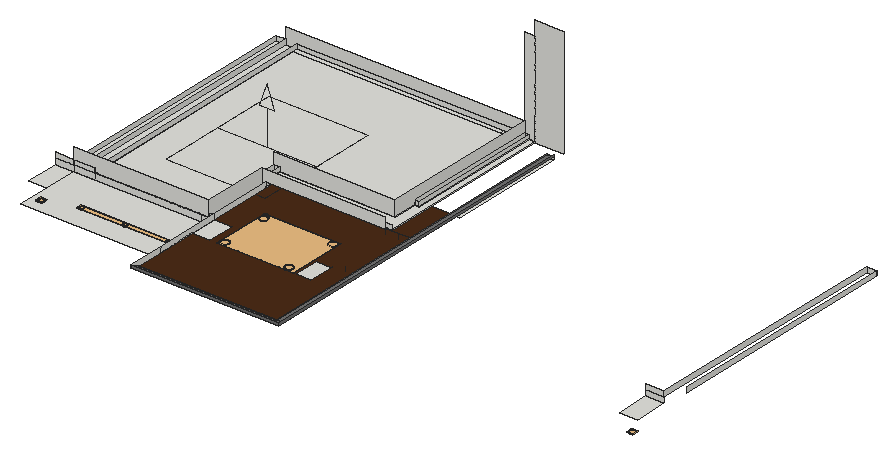
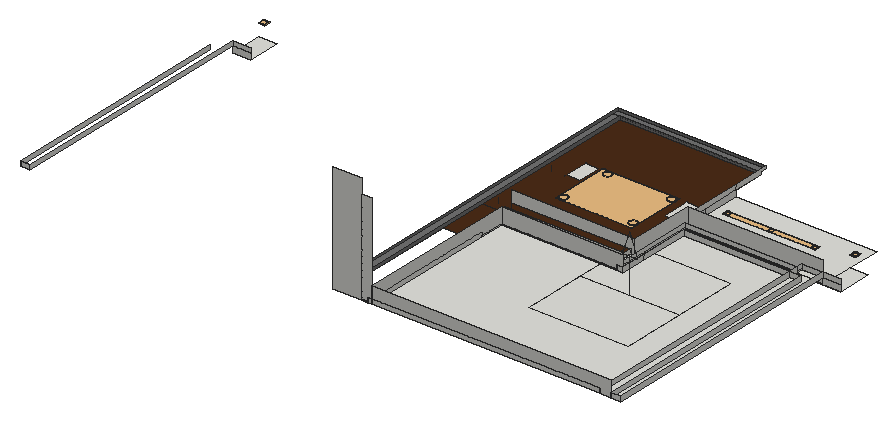
# SketchUp Ruby script. Lengths in inches.
U = 1.inch
M = Sketchup.active_model
def pt(a) = Geom::Point3d.new(a.map { |v| v * U })
def face(e, loops, mat)
  f = e.add_face(loops[0].map { |a| pt(a) })
  loops[1..].each { |l| e.add_face(l.map { |a| pt(a) }).erase! }
  f.material = f.back_material = mat if mat
  f
end
# faces: each face lists its corners as indices into pts; further lists are holes
def faces(e, pts, list, mat = nil) = list.each { |f| face(e, (f[0].is_a?(Array) ? f : [f]).map { |l| l.map { |i| pts[i] } }, mat) }
# xy, xz, yz: faces in a plane at the given z, y or x. An outline is a flat list of corners, or four numbers for a rectangle; further outlines are holes
def ring(l) = l.size == 4 ? [[l[0], l[1]], [l[2], l[1]], [l[2], l[3]], [l[0], l[3]]] : l.each_slice(2).to_a
def flat(e, list, mat, &to3) = list.each { |f| face(e, (f[0].is_a?(Array) ? f : [f]).map { |l| ring(l).map { |u, v| to3.(u, v) } }, mat) }
def xy(e, z, list, mat = nil) = flat(e, list, mat) { |x, y| [x, y, z] }
def xz(e, y, list, mat = nil) = flat(e, list, mat) { |x, z| [x, y, z] }
def yz(e, x, list, mat = nil) = flat(e, list, mat) { |y, z| [x, y, z] }
def lines(e, pts, list) = list.each { |a, b| e.add_line(pt(pts[a]), pt(pts[b])) }
# prism: a flat outline (further loops are holes) pulled along v
def prism(e, loops, v, mat = nil)
  f = face(e, loops, mat); d = Geom::Vector3d.new(v.map { |x| x * U })
  f.pushpull(f.normal.samedirection?(d) ? d.length : -d.length)
end
def box(e, o, s, mat = nil) = prism(e, [[o, [o[0] + s[0], o[1], o[2]], [o[0] + s[0], o[1] + s[1], o[2]], [o[0], o[1] + s[1], o[2]]]], [0, 0, s[2]], mat)
def at(x, y, z, deg = 0) = Geom::Transformation.translation(pt([x, y, z])) * Geom::Transformation.rotation(ORIGIN, Z_AXIS, deg.degrees)
def axes(o, x, y, z) = Geom::Transformation.new([*x, 0, *y, 0, *z, 0, *pt(o).to_a, 1])
def part(name) = M.definitions.add(name)
# library, detail: a bought-in or finely detailed component or shape, given as its bounding box
def library(name, o, s) = part(name).tap { |d| box(d.entities, o, s) }
def detail(e, o, s) = box(e.add_group.entities, o, s)
def put(e, d, t, mat = nil) = e.add_instance(d, t).tap { |i| i.material = mat if mat }
def group(e, t, mat = nil) = e.add_group.tap { |g| g.transformation = t; g.material = mat if mat }.entities
root = M.entities
M.materials.add("[Color M05]").color = [114, 114, 114]
M.materials.add("[Wood Veneer 01]").color = [76, 44, 23]
c1 = library("Group\#26",[-0.5,-0.5,-0.1],[9.125,9.125,0.2])
c2 = library("Group\#20",[-0.5,-0.5,-0.1],[139.5,7.875,0.2])
c3 = library("Group\#21",[-0.5,-0.5,-0.1],[115.36,88.99,0.2])
c4 = part("Group266\#1")
p = [[0,0,0],[0,0,-53.16],[-11.52,0,-53.16],[75.01,-97.09,0],[-75.01,-97.09,0],[75.01,97.09,0],
  [75.01,0,0],[-75.01,97.09,0],[11.52,0,-53.16],[-75.01,0,0],[0,0,-86.05]]
lines(c4.entities,p,[[0,1],[1,2],[3,4],[5,6],[7,5],[1,8],[9,0],[0,6],[8,10],[4,9],[6,3],[2,10],
  [9,7]])
c5 = part("Rectangle Light\#1")
put(c5.entities,c4,at(0,0,0))
xy(root,104.8125,[[252.74,588.74,279.74,638.99],[1145.33,588.74,1172.33,638.99]])
xy(root,104.9375,[[[279.74,538.49,491.71,638.99],[294.3,556.14,295.35,556.28,296.33,556.69,297.18,557.33,297.82,558.17,298.23,559.15,298.37,560.2,298.23,561.26,297.82,562.23,297.18,563.08,296.33,563.72,295.35,564.13,294.3,564.27,293.25,564.13,292.27,563.72,291.43,563.08,290.79,562.23,290.38,561.26,290.24,560.2,290.38,559.15,290.79,558.17,291.43,557.33,292.27,556.69,293.25,556.28],[342.36,572.82,343.25,572.9375,344.08,573.28,344.79,573.83,345.34,574.54,345.68,575.37,345.8,576.26,345.68,577.15,345.34,577.98,344.79,578.6875,344.08,579.23,343.25,579.58,342.36,579.69,341.47,579.58,340.64,579.23,339.93,578.6875,339.38,577.98,339.04,577.15,338.92,576.26,339.04,575.37,339.38,574.54,339.93,573.83,340.64,573.28,341.47,572.9375],[408.17,572.82,409.0625,572.9375,409.89,573.28,410.6,573.83,411.15,574.54,411.49,575.37,411.61,576.26,411.49,577.15,411.15,577.98,410.6,578.6875,409.89,579.23,409.0625,579.58,408.17,579.69,407.28,579.58,406.45,579.23,405.74,578.6875,405.2,577.98,404.85,577.15,404.74,576.26,404.85,575.37,405.2,574.54,405.74,573.83,406.45,573.28,407.28,572.9375],[473.99,572.82,474.875,572.9375,475.7,573.28,476.42,573.83,476.96,574.54,477.31,575.37,477.42,576.26,477.31,577.15,476.96,577.98,476.42,578.6875,475.7,579.23,474.875,579.58,473.99,579.69,473.1,579.58,472.27,579.23,471.55,578.6875,471.01,577.98,470.66,577.15,470.55,576.26,470.66,575.37,471.01,574.54,471.55,573.83,472.27,573.28,473.1,572.9375]]])
xy(root,113.8125,[[491.71,597.99,519.14,638.93],[649.86,597.99,671.36,635.56],[279.74,638.99,312.05,648.22],[312.05,638.99,472.88,648.22],[279.74,648.22,312.05,648.22,312.05,662.52,294.47,662.52,294.47,1021.31,279.74,1021.31],
  [294.47,662.52,312.05,1021.31],[312.05,662.52,312.05,1013.93,655.66,1013.93,655.66,776.62,471.68,776.62,471.68,662.52],[662.14,749.87,671.36,1021.31],[704.8,824.85,715.11,1001.66],[312.05,1013.93,624.8,1021.31],
  [624.8,1013.93,655.66,1021.31]])
xy(root,113.8125,[[[491.71,491.12,491.71,597.99,519.14,597.99,519.14,638.93,491.71,638.93,491.71,749.87,704.8,749.87,704.8,491.12],[649.86,597.99,671.36,635.56],[633.34,598.1875,634.9,598.39,636.34,598.99,637.58,599.94,638.54,601.1875,639.14,602.63,639.34,604.1875,639.14,605.74,638.54,607.1875,637.58,608.43,636.34,609.38,634.9,609.98,633.34,610.1875,631.79,609.98,630.34,609.38,629.1,608.43,628.15,607.1875,627.55,605.74,627.34,604.1875,627.55,602.63,628.15,601.1875,629.1,599.94,630.34,598.99,631.79,598.39],[536.53,670.9375,538.08,671.14,539.53,671.74,540.77,672.69,541.73,673.9375,542.33,675.38,542.53,676.9375,542.33,678.49,541.73,679.9375,540.77,681.18,539.53,682.13,538.08,682.73,536.53,682.9375,534.98,682.73,533.53,682.13,532.29,681.18,531.33,679.9375,530.73,678.49,530.53,676.9375,530.73,675.38,531.33,673.9375,532.29,672.69,533.53,671.74,534.98,671.14],[536.53,598.1875,538.08,598.39,539.53,598.99,540.77,599.94,541.73,601.1875,542.33,602.63,542.53,604.1875,542.33,605.74,541.73,607.1875,540.77,608.43,539.53,609.38,538.08,609.98,536.53,610.1875,534.98,609.98,533.53,609.38,532.29,608.43,531.33,607.1875,530.73,605.74,530.53,604.1875,530.73,602.63,531.33,601.1875,532.29,599.94,533.53,598.99,534.98,598.39],[638.89,674.17,640.44,674.38,641.89,674.98,643.13,675.93,644.09,677.17,644.6875,678.62,644.89,680.17,644.6875,681.73,644.09,683.17,643.13,684.42,641.89,685.37,640.44,685.97,638.89,686.17,637.34,685.97,635.89,685.37,634.65,684.42,633.7,683.17,633.1,681.73,632.89,680.17,633.1,678.62,633.7,677.17,634.65,675.93,635.89,674.98,637.34,674.38]],[671.36,749.87,704.8,824.85]],"[Wood Veneer 01]")
xy(root,115.0625,[[312.05,638.99,484.3,638.99,484.3,738.06,491.71,738.06,491.71,749.87,671.36,749.87,671.36,1021.31,662.14,1021.31,662.14,813.85,655.66,813.85,655.66,776.62,481.36,776.62,481.36,648.22,312.05,648.22]])
xy(root,118.1875,[[491.71,481.81,715.11,491.12],[704.8,491.12,715.11,1001.66]],"[Color M05]")
xz(root,481.81,[[491.71,118.1875,715.11,121.3125]],"[Color M05]")
xz(root,491.12,[[491.71,113.8125,704.8,118.1875]],"[Color M05]")
xz(root,638.99,[[252.74,104.8125,279.74,113.8125],[279.74,104.8125,312.05,104.9375],[1145.33,104.8125,1172.33,113.8125],[279.74,104.9375,312.05,113.8125],[312.05,104.9375,472.88,113.8125],
  [472.88,104.9375,491.71,113.8125],[252.74,113.8125,279.74,121.3125],[279.74,113.8125,312.05,121.3125],[312.05,113.8125,484.3,115.0625],[484.3,113.8125,491.71,121.3125],
  [1145.33,113.8125,1172.33,121.3125],[312.05,115.0625,484.3,115.0625,484.3,138.1875,279.74,138.1875,279.74,121.3125,312.05,121.3125]])
xz(root,648.22,[[312.05,113.8125,481.36,115.0625],[312.05,115.0625,481.36,121.3125]])
xz(root,662.52,[[294.47,113.8125,471.68,121.3125]])
xz(root,738.06,[[484.3,113.8125,491.71,115.0625],[484.3,115.0625,491.71,115.0625,491.71,121.3125,671.36,121.3125,671.36,138.1875,484.3,138.1875]])
xz(root,749.87,[[491.71,113.8125,662.14,115.0625],[662.14,113.8125,671.36,115.0625],[491.71,115.0625,671.36,121.3125]])
xz(root,776.62,[[471.68,113.8125,481.36,121.3125],[481.36,113.8125,655.66,115.0625],[481.36,115.0625,655.66,115.0625,655.66,138.1875,471.68,138.1875,471.68,121.3125,481.36,121.3125]])
xz(root,813.85,[[655.66,113.8125,662.14,115.0625],[655.66,115.0625,662.14,121.3125]])
xz(root,1001.66,[[704.8,113.8125,715.11,118.1875]])
xz(root,1021.31,[[279.74,113.8125,294.47,121.3125],[294.47,113.8125,294.47,138.1875,655.66,138.1875,655.66,121.3125,312.05,121.3125,312.05,113.8125],[312.05,113.8125,655.66,121.3125],[655.66,113.8125,662.14,121.3125],[662.14,113.8125,671.36,115.0625],
  [671.36,113.8125,715.11,279.25],[1172.33,113.8125,1187.0625,121.3125],[662.14,115.0625,662.14,121.3125,655.66,121.3125,655.66,258.1875,671.36,258.1875,671.36,115.0625]])
yz(root,279.74,[[638.99,113.8125,1021.31,121.3125]])
yz(root,294.47,[[662.52,113.8125,1021.31,121.3125]])
yz(root,312.05,[[638.99,113.8125,648.22,115.0625],[648.22,113.8125,1021.31,121.3125],[638.99,115.0625,648.22,121.3125]])
yz(root,471.68,[[662.52,113.8125,738.06,121.3125],[738.06,113.8125,776.62,121.3125]])
yz(root,481.36,[[648.22,113.8125,776.62,115.0625],[648.22,115.0625,776.62,121.3125]])
yz(root,484.3,[[638.99,113.8125,738.06,115.0625],[638.99,115.0625,738.06,138.1875]])
yz(root,491.71,[[538.49,104.9375,597.99,113.8125],[597.99,104.9375,638.93,113.8125],[638.93,104.9375,638.99,113.8125],[491.12,113.8125,491.12,118.1875,481.81,118.1875,481.81,121.3125,538.49,121.3125,538.49,113.8125],[538.49,113.8125,638.99,121.3125],
  [638.99,113.8125,738.06,121.3125],[738.06,113.8125,749.87,115.0625],[738.06,115.0625,749.87,121.3125]])
yz(root,655.66,[[776.62,113.8125,813.85,115.0625],[813.85,113.8125,1021.31,121.3125],[776.62,115.0625,813.85,115.0625,813.85,121.3125,1021.31,121.3125,1021.31,138.1875,776.62,138.1875]])
yz(root,662.14,[[813.85,113.8125,1021.31,115.0625],[813.85,115.0625,1021.31,121.3125]])
yz(root,671.36,[[749.87,113.8125,1021.31,115.0625]])
yz(root,704.8,[[491.12,113.8125,1001.66,118.1875]],"[Color M05]")
yz(root,715.11,[[481.81,118.1875,1001.66,121.3125]],"[Color M05]")
yz(root,1172.33,[[638.99,113.8125,1021.31,121.3125]])
yz(root,1187.0625,[[662.52,113.8125,1021.31,121.3125]])
p = [[294.3,556.14,104.9375],[293.25,556.28,104.9375],[293.25,556.28,105.875],[294.3,556.14,105.875],[295.35,556.28,104.9375],[295.35,556.28,105.875],
  [1186.89,556.14,104.9375],[1185.84,556.28,104.9375],[1185.84,556.28,105.875],[1186.89,556.14,105.875],[292.27,556.69,104.9375],[292.27,556.69,105.875],
  [296.33,556.69,104.9375],[296.33,556.69,105.875],[1184.86,556.69,104.9375],[1184.86,556.69,105.875],[291.43,557.33,104.9375],[291.43,557.33,105.875],
  [297.18,557.33,104.9375],[297.18,557.33,105.875],[1184.02,557.33,104.9375],[1184.02,557.33,105.875],[290.79,558.17,104.9375],[290.79,558.17,105.875],
  [297.82,558.17,104.9375],[297.82,558.17,105.875],[1183.375,558.17,104.9375],[1183.375,558.17,105.875],[290.38,559.15,104.9375],[290.38,559.15,105.875],
  [298.23,559.15,104.9375],[298.23,559.15,105.875],[1182.97,559.15,104.9375],[1182.97,559.15,105.875],[290.24,560.2,104.9375],[290.24,560.2,105.875],
  [298.37,560.2,104.9375],[298.37,560.2,105.875],[1182.83,560.2,104.9375],[1182.83,560.2,105.875],[290.38,561.26,104.9375],[290.38,561.26,105.875],
  [298.23,561.26,104.9375],[298.23,561.26,105.875],[1182.97,561.26,104.9375],[1182.97,561.26,105.875],[290.79,562.23,104.9375],[290.79,562.23,105.875],
  [297.82,562.23,104.9375],[297.82,562.23,105.875],[1183.375,562.23,104.9375],[1183.375,562.23,105.875],[291.43,563.08,104.9375],[291.43,563.08,105.875],
  [297.18,563.08,104.9375],[297.18,563.08,105.875],[1184.02,563.08,104.9375],[1184.02,563.08,105.875],[292.27,563.72,104.9375],[292.27,563.72,105.875],
  [296.33,563.72,104.9375],[296.33,563.72,105.875],[1184.86,563.72,104.9375],[1184.86,563.72,105.875],[293.25,564.13,104.9375],[293.25,564.13,105.875],
  [295.35,564.13,104.9375],[295.35,564.13,105.875],[1185.84,564.13,104.9375],[1185.84,564.13,105.875],[294.3,564.27,104.9375],[294.3,564.27,105.875],
  [1186.89,564.27,104.9375],[1186.89,564.27,105.875],[342.36,572.82,104.9375],[341.47,572.9375,104.9375],[341.47,572.9375,105.375],[342.36,572.82,105.375],
  [343.25,572.9375,104.9375],[343.25,572.9375,105.375],[408.17,572.82,104.9375],[407.28,572.9375,104.9375],[407.28,572.9375,105.375],[408.17,572.82,105.375],
  [409.0625,572.9375,104.9375],[409.0625,572.9375,105.375],[473.99,572.82,104.9375],[473.1,572.9375,104.9375],[473.1,572.9375,105.375],[473.99,572.82,105.375],
  [474.875,572.9375,104.9375],[474.875,572.9375,105.375],[340.64,573.28,104.9375],[340.64,573.28,105.375],[344.08,573.28,104.9375],[344.08,573.28,105.375],
  [406.45,573.28,104.9375],[406.45,573.28,105.375],[409.89,573.28,104.9375],[409.89,573.28,105.375],[472.27,573.28,104.9375],[472.27,573.28,105.375],
  [475.7,573.28,104.9375],[475.7,573.28,105.375],[339.93,573.83,104.9375],[339.93,573.83,105.375],[344.79,573.83,104.9375],[344.79,573.83,105.375],
  [405.74,573.83,104.9375],[405.74,573.83,105.375],[410.6,573.83,104.9375],[410.6,573.83,105.375],[471.55,573.83,104.9375],[471.55,573.83,105.375],
  [476.42,573.83,104.9375],[476.42,573.83,105.375],[339.38,574.54,104.9375],[339.38,574.54,105.375],[345.34,574.54,104.9375],[345.34,574.54,105.375],
  [405.2,574.54,104.9375],[405.2,574.54,105.375],[411.15,574.54,104.9375],[411.15,574.54,105.375],[471.01,574.54,104.9375],[471.01,574.54,105.375],
  [476.96,574.54,104.9375],[476.96,574.54,105.375],[339.04,575.37,104.9375],[339.04,575.37,105.375],[345.68,575.37,104.9375],[345.68,575.37,105.375],
  [404.85,575.37,104.9375],[404.85,575.37,105.375],[411.49,575.37,104.9375],[411.49,575.37,105.375],[470.66,575.37,104.9375],[470.66,575.37,105.375],
  [477.31,575.37,104.9375],[477.31,575.37,105.375],[338.92,576.26,104.9375],[338.92,576.26,105.375],[345.8,576.26,104.9375],[345.8,576.26,105.375],
  [404.74,576.26,104.9375],[404.74,576.26,105.375],[411.61,576.26,104.9375],[411.61,576.26,105.375],[470.55,576.26,104.9375],[470.55,576.26,105.375],
  [477.42,576.26,104.9375],[477.42,576.26,105.375],[339.04,577.15,104.9375],[339.04,577.15,105.375],[345.68,577.15,104.9375],[345.68,577.15,105.375],
  [404.85,577.15,104.9375],[404.85,577.15,105.375],[411.49,577.15,104.9375],[411.49,577.15,105.375],[470.66,577.15,104.9375],[470.66,577.15,105.375],
  [477.31,577.15,104.9375],[477.31,577.15,105.375],[339.38,577.98,104.9375],[339.38,577.98,105.375],[345.34,577.98,104.9375],[345.34,577.98,105.375],
  [405.2,577.98,104.9375],[405.2,577.98,105.375],[411.15,577.98,104.9375],[411.15,577.98,105.375],[471.01,577.98,104.9375],[471.01,577.98,105.375],
  [476.96,577.98,104.9375],[476.96,577.98,105.375],[339.93,578.6875,104.9375],[339.93,578.6875,105.375],[344.79,578.6875,104.9375],[344.79,578.6875,105.375],
  [405.74,578.6875,104.9375],[405.74,578.6875,105.375],[410.6,578.6875,104.9375],[410.6,578.6875,105.375],[471.55,578.6875,104.9375],[471.55,578.6875,105.375],
  [476.42,578.6875,104.9375],[476.42,578.6875,105.375],[340.64,579.23,104.9375],[340.64,579.23,105.375],[344.08,579.23,104.9375],[344.08,579.23,105.375],
  [406.45,579.23,104.9375],[406.45,579.23,105.375],[409.89,579.23,104.9375],[409.89,579.23,105.375],[472.27,579.23,104.9375],[472.27,579.23,105.375],
  [475.7,579.23,104.9375],[475.7,579.23,105.375],[341.47,579.58,104.9375],[341.47,579.58,105.375],[343.25,579.58,104.9375],[343.25,579.58,105.375],
  [407.28,579.58,104.9375],[407.28,579.58,105.375],[409.0625,579.58,104.9375],[409.0625,579.58,105.375],[473.1,579.58,104.9375],[473.1,579.58,105.375],
  [474.875,579.58,104.9375],[474.875,579.58,105.375],[342.36,579.69,104.9375],[342.36,579.69,105.375],[408.17,579.69,104.9375],[408.17,579.69,105.375],
  [473.99,579.69,104.9375],[473.99,579.69,105.375],[536.53,598.1875,113.8125],[534.98,598.39,113.8125],[534.98,598.39,114.6875],[536.53,598.1875,114.6875],
  [538.08,598.39,113.8125],[538.08,598.39,114.6875],[633.34,598.1875,113.8125],[631.79,598.39,113.8125],[631.79,598.39,114.6875],[633.34,598.1875,114.6875],
  [634.9,598.39,113.8125],[634.9,598.39,114.6875],[533.53,598.99,113.8125],[533.53,598.99,114.6875],[539.53,598.99,113.8125],[539.53,598.99,114.6875],
  [630.34,598.99,113.8125],[630.34,598.99,114.6875],[636.34,598.99,113.8125],[636.34,598.99,114.6875],[532.29,599.94,113.8125],[532.29,599.94,114.6875],
  [540.77,599.94,113.8125],[540.77,599.94,114.6875],[629.1,599.94,113.8125],[629.1,599.94,114.6875],[637.58,599.94,113.8125],[637.58,599.94,114.6875],
  [531.33,601.1875,113.8125],[531.33,601.1875,114.6875],[541.73,601.1875,113.8125],[541.73,601.1875,114.6875],[628.15,601.1875,113.8125],[628.15,601.1875,114.6875],
  [638.54,601.1875,113.8125],[638.54,601.1875,114.6875],[530.73,602.63,113.8125],[530.73,602.63,114.6875],[542.33,602.63,113.8125],[542.33,602.63,114.6875],
  [627.55,602.63,113.8125],[627.55,602.63,114.6875],[639.14,602.63,113.8125],[639.14,602.63,114.6875],[530.53,604.1875,113.8125],[530.53,604.1875,114.6875],
  [542.53,604.1875,113.8125],[542.53,604.1875,114.6875],[627.34,604.1875,113.8125],[627.34,604.1875,114.6875],[639.34,604.1875,113.8125],[639.34,604.1875,114.6875],
  [530.73,605.74,113.8125],[530.73,605.74,114.6875],[542.33,605.74,113.8125],[542.33,605.74,114.6875],[627.55,605.74,113.8125],[627.55,605.74,114.6875],
  [639.14,605.74,113.8125],[639.14,605.74,114.6875],[531.33,607.1875,113.8125],[531.33,607.1875,114.6875],[541.73,607.1875,113.8125],[541.73,607.1875,114.6875],
  [628.15,607.1875,113.8125],[628.15,607.1875,114.6875],[638.54,607.1875,113.8125],[638.54,607.1875,114.6875],[532.29,608.43,113.8125],[532.29,608.43,114.6875],
  [540.77,608.43,113.8125],[540.77,608.43,114.6875],[629.1,608.43,113.8125],[629.1,608.43,114.6875],[637.58,608.43,113.8125],[637.58,608.43,114.6875],
  [533.53,609.38,113.8125],[533.53,609.38,114.6875],[539.53,609.38,113.8125],[539.53,609.38,114.6875],[630.34,609.38,113.8125],[630.34,609.38,114.6875],
  [636.34,609.38,113.8125],[636.34,609.38,114.6875],[534.98,609.98,113.8125],[534.98,609.98,114.6875],[538.08,609.98,113.8125],[538.08,609.98,114.6875],
  [631.79,609.98,113.8125],[631.79,609.98,114.6875],[634.9,609.98,113.8125],[634.9,609.98,114.6875],[536.53,610.1875,113.8125],[536.53,610.1875,114.6875],
  [633.34,610.1875,113.8125],[633.34,610.1875,114.6875],[536.53,670.9375,113.8125],[534.98,671.14,113.8125],[534.98,671.14,114.6875],[536.53,670.9375,114.6875],
  [538.08,671.14,113.8125],[538.08,671.14,114.6875],[533.53,671.74,113.8125],[533.53,671.74,114.6875],[539.53,671.74,113.8125],[539.53,671.74,114.6875],
  [532.29,672.69,113.8125],[532.29,672.69,114.6875],[540.77,672.69,113.8125],[540.77,672.69,114.6875],[531.33,673.9375,113.8125],[531.33,673.9375,114.6875],
  [541.73,673.9375,113.8125],[541.73,673.9375,114.6875],[530.73,675.38,113.8125],[530.73,675.38,114.6875],[542.33,675.38,113.8125],[542.33,675.38,114.6875],
  [638.89,674.17,113.8125],[637.34,674.38,113.8125],[637.34,674.38,114.6875],[638.89,674.17,114.6875],[640.44,674.38,113.8125],[640.44,674.38,114.6875],
  [635.89,674.98,113.8125],[635.89,674.98,114.6875],[641.89,674.98,113.8125],[641.89,674.98,114.6875],[634.65,675.93,113.8125],[634.65,675.93,114.6875],
  [643.13,675.93,113.8125],[643.13,675.93,114.6875],[530.53,676.9375,113.8125],[530.53,676.9375,114.6875],[542.53,676.9375,113.8125],[542.53,676.9375,114.6875],
  [633.7,677.17,113.8125],[633.7,677.17,114.6875],[644.09,677.17,113.8125],[644.09,677.17,114.6875],[530.73,678.49,113.8125],[530.73,678.49,114.6875],
  [542.33,678.49,113.8125],[542.33,678.49,114.6875],[633.1,678.62,113.8125],[633.1,678.62,114.6875],[644.6875,678.62,113.8125],[644.6875,678.62,114.6875],
  [531.33,679.9375,113.8125],[531.33,679.9375,114.6875],[541.73,679.9375,113.8125],[541.73,679.9375,114.6875],[632.89,680.17,113.8125],[632.89,680.17,114.6875],
  [644.89,680.17,113.8125],[644.89,680.17,114.6875],[532.29,681.18,113.8125],[532.29,681.18,114.6875],[540.77,681.18,113.8125],[540.77,681.18,114.6875],
  [633.1,681.73,113.8125],[633.1,681.73,114.6875],[644.6875,681.73,113.8125],[644.6875,681.73,114.6875],[533.53,682.13,113.8125],[533.53,682.13,114.6875],
  [539.53,682.13,113.8125],[539.53,682.13,114.6875],[633.7,683.17,113.8125],[633.7,683.17,114.6875],[644.09,683.17,113.8125],[644.09,683.17,114.6875],
  [534.98,682.73,113.8125],[534.98,682.73,114.6875],[538.08,682.73,113.8125],[538.08,682.73,114.6875],[536.53,682.9375,113.8125],[536.53,682.9375,114.6875],
  [634.65,684.42,113.8125],[634.65,684.42,114.6875],[643.13,684.42,113.8125],[643.13,684.42,114.6875],[635.89,685.37,113.8125],[635.89,685.37,114.6875],
  [641.89,685.37,113.8125],[641.89,685.37,114.6875],[637.34,685.97,113.8125],[637.34,685.97,114.6875],[640.44,685.97,113.8125],[640.44,685.97,114.6875],
  [638.89,686.17,113.8125],[638.89,686.17,114.6875],[671.36,638.93,113.8125],[671.36,635.56,113.8125],[690.8,638.99,113.8125],[690.8,638.99,121.3125],
  [690.8,638.93,113.8125],[690.8,738.06,121.3125],[690.8,738.06,113.8125],[671.36,738.06,121.3125],[671.36,738.06,113.8125]]
faces(root,p,[[0,1,2,3],[4,0,3,5],[6,7,8,9],[1,10,11,2],[12,4,5,13],[7,14,15,8],[10,16,17,11],[18,12,13,19],
  [14,20,21,15],[16,22,23,17],[24,18,19,25],[20,26,27,21],[22,28,29,23],[30,24,25,31],[26,32,33,27],[28,34,35,29],
  [36,30,31,37],[32,38,39,33],[34,40,41,35],[42,36,37,43],[38,44,45,39],[40,46,47,41],[48,42,43,49],[44,50,51,45],
  [46,52,53,47],[54,48,49,55],[50,56,57,51],[52,58,59,53],[60,54,55,61],[56,62,63,57],[58,64,65,59],[66,60,61,67],
  [62,68,69,63],[64,70,71,65],[70,66,67,71],[68,72,73,69],[74,75,76,77],[78,74,77,79],[80,81,82,83],[84,80,83,85],
  [86,87,88,89],[90,86,89,91],[75,92,93,76],[94,78,79,95],[81,96,97,82],[98,84,85,99],[87,100,101,88],[102,90,91,103],
  [92,104,105,93],[106,94,95,107],[96,108,109,97],[110,98,99,111],[100,112,113,101],[114,102,103,115],[104,116,117,105],[118,106,107,119],
  [108,120,121,109],[122,110,111,123],[112,124,125,113],[126,114,115,127],[116,128,129,117],[130,118,119,131],[120,132,133,121],[134,122,123,135],
  [124,136,137,125],[138,126,127,139],[128,140,141,129],[142,130,131,143],[132,144,145,133],[146,134,135,147],[136,148,149,137],[150,138,139,151],
  [140,152,153,141],[154,142,143,155],[144,156,157,145],[158,146,147,159],[148,160,161,149],[162,150,151,163],[152,164,165,153],[166,154,155,167],
  [156,168,169,157],[170,158,159,171],[160,172,173,161],[174,162,163,175],[164,176,177,165],[178,166,167,179],[168,180,181,169],[182,170,171,183],
  [172,184,185,173],[186,174,175,187],[176,188,189,177],[190,178,179,191],[180,192,193,181],[194,182,183,195],[184,196,197,185],[198,186,187,199],
  [188,200,201,189],[202,190,191,203],[192,204,205,193],[206,194,195,207],[196,208,209,197],[210,198,199,211],[200,212,213,201],[212,202,203,213],
  [204,214,215,205],[214,206,207,215],[208,216,217,209],[216,210,211,217]])
faces(root,p,[[218,219,220,221],[222,218,221,223],[224,225,226,227],[228,224,227,229],[219,230,231,220],[232,222,223,233],[225,234,235,226],[236,228,229,237],
  [230,238,239,231],[240,232,233,241],[234,242,243,235],[244,236,237,245],[238,246,247,239],[248,240,241,249],[242,250,251,243],[252,244,245,253],
  [246,254,255,247],[256,248,249,257],[250,258,259,251],[260,252,253,261],[254,262,263,255],[264,256,257,265],[258,266,267,259],[268,260,261,269],
  [262,270,271,263],[272,264,265,273],[266,274,275,267],[276,268,269,277],[270,278,279,271],[280,272,273,281],[274,282,283,275],[284,276,277,285],
  [278,286,287,279],[288,280,281,289],[282,290,291,283],[292,284,285,293],[286,294,295,287],[296,288,289,297],[290,298,299,291],[300,292,293,301],
  [294,302,303,295],[304,296,297,305],[298,306,307,299],[308,300,301,309],[302,310,311,303],[310,304,305,311],[306,312,313,307],[312,308,309,313],
  [314,315,316,317],[318,314,317,319],[315,320,321,316],[322,318,319,323],[320,324,325,321],[326,322,323,327],[324,328,329,325],[330,326,327,331],
  [328,332,333,329],[334,330,331,335],[336,337,338,339],[340,336,339,341],[337,342,343,338],[344,340,341,345],[342,346,347,343],[348,344,345,349],
  [332,350,351,333],[352,334,335,353],[346,354,355,347],[356,348,349,357],[350,358,359,351],[360,352,353,361],[354,362,363,355],[364,356,357,365],
  [358,366,367,359],[368,360,361,369],[362,370,371,363],[372,364,365,373],[366,374,375,367],[376,368,369,377],[370,378,379,371],[380,372,373,381],
  [374,382,383,375],[384,376,377,385],[378,386,387,379],[388,380,381,389],[382,390,391,383],[392,384,385,393],[390,394,395,391],[394,392,393,395],
  [386,396,397,387],[398,388,389,399],[396,400,401,397],[402,398,399,403],[400,404,405,401],[406,402,403,407],[404,408,409,405],[408,406,407,409]],"[Wood Veneer 01]")
lines(root,p,[[410,411],[412,413],[412,414],[415,416],[417,418]])
put(root,c1,at(1182.83,556.14,105.875))
put(root,c1,at(290.24,556.14,105.875))
put(root,c2,at(338.92,572.82,105.375))
put(root,c3,at(530.53,598.1875,114.6875))
put(root,c5,axes([431.33,814.73,113.82],[1,0,0],[0,1,0],[0,0,-1]))
